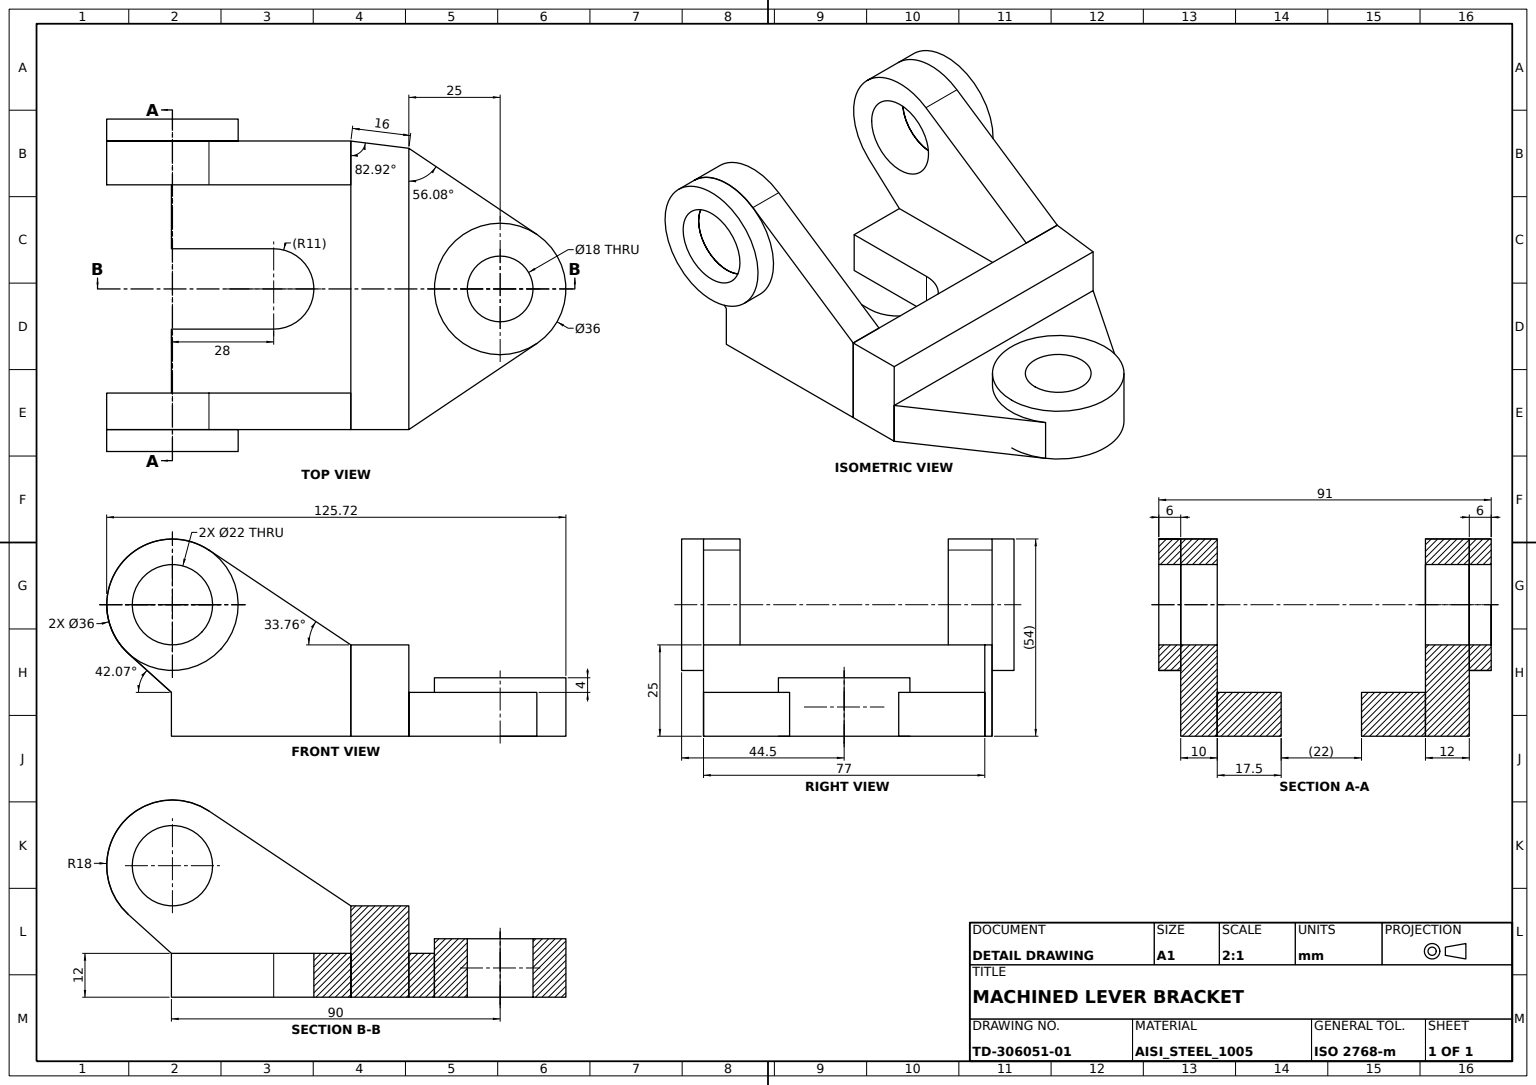
ISO-10303-21;
HEADER;
FILE_DESCRIPTION((''),'2;1');
FILE_NAME('','',(''),(''),'','','');
FILE_SCHEMA(('AUTOMOTIVE_DESIGN'));
ENDSEC;
DATA;
#1=APPLICATION_CONTEXT('');
#2=PRODUCT_CONTEXT('',#1,'mechanical');
#3=PRODUCT('','','',(#2));
#4=PRODUCT_DEFINITION_FORMATION('','',#3);
#5=PRODUCT_DEFINITION_CONTEXT('',#1,'design');
#6=PRODUCT_DEFINITION('','',#4,#5);
#7=PRODUCT_DEFINITION_SHAPE('','',#6);
#8=(LENGTH_UNIT()NAMED_UNIT(*)SI_UNIT(.MILLI.,.METRE.));
#9=(NAMED_UNIT(*)PLANE_ANGLE_UNIT()SI_UNIT($,.RADIAN.));
#10=(NAMED_UNIT(*)SI_UNIT($,.STERADIAN.)SOLID_ANGLE_UNIT());
#11=UNCERTAINTY_MEASURE_WITH_UNIT(LENGTH_MEASURE(0.005),#8,'distance_accuracy_value','');
#12=(GEOMETRIC_REPRESENTATION_CONTEXT(3)GLOBAL_UNCERTAINTY_ASSIGNED_CONTEXT((#11))GLOBAL_UNIT_ASSIGNED_CONTEXT((#8,#9,#10))REPRESENTATION_CONTEXT('',''));
#13=CARTESIAN_POINT('',(-28.5,-40.877865,-8.));
#14=VERTEX_POINT('',#13);
#15=CARTESIAN_POINT('',(-28.5,-90.,-8.));
#16=VERTEX_POINT('',#15);
#17=DIRECTION('',(0.,-1.,0.));
#18=VECTOR('',#17,1000.);
#19=LINE('',#13,#18);
#20=EDGE_CURVE('',#14,#16,#19,.T.);
#21=ORIENTED_EDGE('',*,*,#20,.T.);
#22=CARTESIAN_POINT('',(-40.5,-90.,-8.));
#23=VERTEX_POINT('',#22);
#24=DIRECTION('',(1.,0.,0.));
#25=VECTOR('',#24,1000.);
#26=LINE('',#22,#25);
#27=EDGE_CURVE('',#23,#16,#26,.T.);
#28=ORIENTED_EDGE('',*,*,#27,.F.);
#29=CARTESIAN_POINT('',(-40.5,-40.877865,-8.));
#30=VERTEX_POINT('',#29);
#31=LINE('',#29,#18);
#32=EDGE_CURVE('',#30,#23,#31,.T.);
#33=ORIENTED_EDGE('',*,*,#32,.F.);
#34=LINE('',#29,#25);
#35=EDGE_CURVE('',#30,#14,#34,.T.);
#36=ORIENTED_EDGE('',*,*,#35,.T.);
#37=EDGE_LOOP('',(#21,#28,#33,#36));
#38=FACE_BOUND('',#37,.T.);
#39=DIRECTION('',(0.,0.,1.));
#40=AXIS2_PLACEMENT_3D('',#29,#39,#17);
#41=PLANE('',#40);
#42=ADVANCED_FACE('',(#38),#41,.F.);
#43=CARTESIAN_POINT('',(-40.5,-90.,4.));
#44=VERTEX_POINT('',#43);
#45=VECTOR('',#39,1000.);
#46=LINE('',#22,#45);
#47=EDGE_CURVE('',#23,#44,#46,.T.);
#48=ORIENTED_EDGE('',*,*,#47,.F.);
#49=ORIENTED_EDGE('',*,*,#27,.T.);
#50=CARTESIAN_POINT('',(-28.5,-90.,4.));
#51=VERTEX_POINT('',#50);
#52=LINE('',#15,#45);
#53=EDGE_CURVE('',#16,#51,#52,.T.);
#54=ORIENTED_EDGE('',*,*,#53,.T.);
#55=LINE('',#43,#25);
#56=EDGE_CURVE('',#44,#51,#55,.T.);
#57=ORIENTED_EDGE('',*,*,#56,.F.);
#58=EDGE_LOOP('',(#48,#49,#54,#57));
#59=FACE_BOUND('',#58,.T.);
#60=DIRECTION('',(0.,1.,0.));
#61=AXIS2_PLACEMENT_3D('',#22,#60,#39);
#62=PLANE('',#61);
#63=ADVANCED_FACE('',(#59),#62,.F.);
#64=ORIENTED_EDGE('',*,*,#53,.F.);
#65=ORIENTED_EDGE('',*,*,#20,.F.);
#66=CARTESIAN_POINT('',(-28.5,-40.877865,17.));
#67=VERTEX_POINT('',#66);
#68=DIRECTION('',(0.,0.,-1.));
#69=VECTOR('',#68,1000.);
#70=LINE('',#66,#69);
#71=EDGE_CURVE('',#67,#14,#70,.T.);
#72=ORIENTED_EDGE('',*,*,#71,.F.);
#73=CARTESIAN_POINT('',(-28.5,-79.720085,42.964502));
#74=VERTEX_POINT('',#73);
#75=DIRECTION('',(0.,0.831361229,-0.555732406));
#76=VECTOR('',#75,1000.);
#77=LINE('',#73,#76);
#78=EDGE_CURVE('',#74,#67,#77,.T.);
#79=ORIENTED_EDGE('',*,*,#78,.F.);
#80=CARTESIAN_POINT('',(-28.5,-101.785016,14.639078));
#81=VERTEX_POINT('',#80);
#82=CARTESIAN_POINT('',(-28.5,-89.723268,28.));
#83=DIRECTION('',(-1.,0.,0.));
#84=AXIS2_PLACEMENT_3D('',#82,#83,#17);
#85=CIRCLE('',#84,18.);
#86=EDGE_CURVE('',#81,#74,#85,.T.);
#87=ORIENTED_EDGE('',*,*,#86,.F.);
#88=DIRECTION('',(0.,-0.742273459,0.670097092));
#89=VECTOR('',#88,1000.);
#90=LINE('',#50,#89);
#91=EDGE_CURVE('',#51,#81,#90,.T.);
#92=ORIENTED_EDGE('',*,*,#91,.F.);
#93=EDGE_LOOP('',(#64,#65,#72,#79,#87,#92));
#94=FACE_BOUND('',#93,.T.);
#95=CARTESIAN_POINT('',(-28.5,-100.723268,28.));
#96=VERTEX_POINT('',#95);
#97=AXIS2_PLACEMENT_3D('',#82,#24,#17);
#98=CIRCLE('',#97,11.);
#99=EDGE_CURVE('',#96,#96,#98,.T.);
#100=ORIENTED_EDGE('',*,*,#99,.F.);
#101=EDGE_LOOP('',(#100));
#102=FACE_BOUND('',#101,.T.);
#103=AXIS2_PLACEMENT_3D('',#82,#83,#39);
#104=PLANE('',#103);
#105=ADVANCED_FACE('',(#94,#102),#104,.F.);
#106=ORIENTED_EDGE('',*,*,#99,.T.);
#107=EDGE_LOOP('',(#106));
#108=FACE_BOUND('',#107,.T.);
#109=CARTESIAN_POINT('',(-40.5,-100.723268,28.));
#110=VERTEX_POINT('',#109);
#111=CARTESIAN_POINT('',(-40.5,-89.723268,28.));
#112=AXIS2_PLACEMENT_3D('',#111,#24,#17);
#113=CIRCLE('',#112,11.);
#114=EDGE_CURVE('',#110,#110,#113,.T.);
#115=ORIENTED_EDGE('',*,*,#114,.F.);
#116=EDGE_LOOP('',(#115));
#117=FACE_BOUND('',#116,.T.);
#118=AXIS2_PLACEMENT_3D('',#111,#24,#68);
#119=CYLINDRICAL_SURFACE('',#118,11.);
#120=ADVANCED_FACE('',(#108,#117),#119,.F.);
#121=ORIENTED_EDGE('',*,*,#114,.T.);
#122=EDGE_LOOP('',(#121));
#123=FACE_BOUND('',#122,.T.);
#124=CARTESIAN_POINT('',(-40.5,-101.785016,14.639078));
#125=VERTEX_POINT('',#124);
#126=CARTESIAN_POINT('',(-40.5,-79.720085,42.964502));
#127=VERTEX_POINT('',#126);
#128=AXIS2_PLACEMENT_3D('',#111,#83,#17);
#129=CIRCLE('',#128,18.);
#130=EDGE_CURVE('',#125,#127,#129,.T.);
#131=ORIENTED_EDGE('',*,*,#130,.T.);
#132=CARTESIAN_POINT('',(-40.5,-40.877865,17.));
#133=VERTEX_POINT('',#132);
#134=LINE('',#126,#76);
#135=EDGE_CURVE('',#127,#133,#134,.T.);
#136=ORIENTED_EDGE('',*,*,#135,.T.);
#137=LINE('',#132,#69);
#138=EDGE_CURVE('',#133,#30,#137,.T.);
#139=ORIENTED_EDGE('',*,*,#138,.T.);
#140=ORIENTED_EDGE('',*,*,#32,.T.);
#141=ORIENTED_EDGE('',*,*,#47,.T.);
#142=LINE('',#43,#89);
#143=EDGE_CURVE('',#44,#125,#142,.T.);
#144=ORIENTED_EDGE('',*,*,#143,.T.);
#145=EDGE_LOOP('',(#131,#136,#139,#140,#141,#144));
#146=FACE_BOUND('',#145,.T.);
#147=AXIS2_PLACEMENT_3D('',#111,#83,#39);
#148=PLANE('',#147);
#149=ADVANCED_FACE('',(#123,#146),#148,.T.);
#150=ORIENTED_EDGE('',*,*,#71,.T.);
#151=ORIENTED_EDGE('',*,*,#35,.F.);
#152=ORIENTED_EDGE('',*,*,#138,.F.);
#153=LINE('',#132,#25);
#154=EDGE_CURVE('',#133,#67,#153,.T.);
#155=ORIENTED_EDGE('',*,*,#154,.T.);
#156=EDGE_LOOP('',(#150,#151,#152,#155));
#157=FACE_BOUND('',#156,.T.);
#158=AXIS2_PLACEMENT_3D('',#132,#17,#68);
#159=PLANE('',#158);
#160=ADVANCED_FACE('',(#157),#159,.F.);
#161=LINE('',#124,#25);
#162=EDGE_CURVE('',#125,#81,#161,.T.);
#163=ORIENTED_EDGE('',*,*,#162,.T.);
#164=ORIENTED_EDGE('',*,*,#86,.T.);
#165=LINE('',#126,#25);
#166=EDGE_CURVE('',#127,#74,#165,.T.);
#167=ORIENTED_EDGE('',*,*,#166,.F.);
#168=ORIENTED_EDGE('',*,*,#130,.F.);
#169=EDGE_LOOP('',(#163,#164,#167,#168));
#170=FACE_BOUND('',#169,.T.);
#171=CYLINDRICAL_SURFACE('',#118,18.);
#172=ADVANCED_FACE('',(#170),#171,.T.);
#173=ORIENTED_EDGE('',*,*,#143,.F.);
#174=ORIENTED_EDGE('',*,*,#56,.T.);
#175=ORIENTED_EDGE('',*,*,#91,.T.);
#176=ORIENTED_EDGE('',*,*,#162,.F.);
#177=EDGE_LOOP('',(#173,#174,#175,#176));
#178=FACE_BOUND('',#177,.T.);
#179=DIRECTION('',(0.,0.670097092,0.742273459));
#180=AXIS2_PLACEMENT_3D('',#43,#179,#88);
#181=PLANE('',#180);
#182=ADVANCED_FACE('',(#178),#181,.F.);
#183=ORIENTED_EDGE('',*,*,#135,.F.);
#184=ORIENTED_EDGE('',*,*,#166,.T.);
#185=ORIENTED_EDGE('',*,*,#78,.T.);
#186=ORIENTED_EDGE('',*,*,#154,.F.);
#187=EDGE_LOOP('',(#183,#184,#185,#186));
#188=FACE_BOUND('',#187,.T.);
#189=DIRECTION('',(0.,-0.555732406,-0.831361229));
#190=AXIS2_PLACEMENT_3D('',#126,#189,#75);
#191=PLANE('',#190);
#192=ADVANCED_FACE('',(#188),#191,.F.);
#193=CLOSED_SHELL('',(#42,#63,#105,#120,#149,#160,#172,#182,#192));
#194=MANIFOLD_SOLID_BREP('',#193);
#195=CARTESIAN_POINT('',(38.5,-78.723268,28.));
#196=VERTEX_POINT('',#195);
#197=CARTESIAN_POINT('',(38.5,-89.723268,28.));
#198=AXIS2_PLACEMENT_3D('',#197,#83,#60);
#199=CIRCLE('',#198,11.);
#200=EDGE_CURVE('',#196,#196,#199,.T.);
#201=ORIENTED_EDGE('',*,*,#200,.F.);
#202=EDGE_LOOP('',(#201));
#203=FACE_BOUND('',#202,.T.);
#204=CARTESIAN_POINT('',(28.5,-78.723268,28.));
#205=VERTEX_POINT('',#204);
#206=CARTESIAN_POINT('',(28.5,-89.723268,28.));
#207=AXIS2_PLACEMENT_3D('',#206,#83,#60);
#208=CIRCLE('',#207,11.);
#209=EDGE_CURVE('',#205,#205,#208,.T.);
#210=ORIENTED_EDGE('',*,*,#209,.T.);
#211=EDGE_LOOP('',(#210));
#212=FACE_BOUND('',#211,.T.);
#213=AXIS2_PLACEMENT_3D('',#197,#83,#39);
#214=CYLINDRICAL_SURFACE('',#213,11.);
#215=ADVANCED_FACE('',(#203,#212),#214,.F.);
#216=CARTESIAN_POINT('',(28.5,-90.,-8.));
#217=VERTEX_POINT('',#216);
#218=CARTESIAN_POINT('',(28.5,-40.877865,-8.));
#219=VERTEX_POINT('',#218);
#220=VECTOR('',#60,1000.);
#221=LINE('',#216,#220);
#222=EDGE_CURVE('',#217,#219,#221,.T.);
#223=ORIENTED_EDGE('',*,*,#222,.T.);
#224=CARTESIAN_POINT('',(38.5,-40.877865,-8.));
#225=VERTEX_POINT('',#224);
#226=VECTOR('',#83,1000.);
#227=LINE('',#224,#226);
#228=EDGE_CURVE('',#225,#219,#227,.T.);
#229=ORIENTED_EDGE('',*,*,#228,.F.);
#230=CARTESIAN_POINT('',(38.5,-90.,-8.));
#231=VERTEX_POINT('',#230);
#232=LINE('',#230,#220);
#233=EDGE_CURVE('',#231,#225,#232,.T.);
#234=ORIENTED_EDGE('',*,*,#233,.F.);
#235=LINE('',#230,#226);
#236=EDGE_CURVE('',#231,#217,#235,.T.);
#237=ORIENTED_EDGE('',*,*,#236,.T.);
#238=EDGE_LOOP('',(#223,#229,#234,#237));
#239=FACE_BOUND('',#238,.T.);
#240=AXIS2_PLACEMENT_3D('',#230,#39,#24);
#241=PLANE('',#240);
#242=ADVANCED_FACE('',(#239),#241,.F.);
#243=CARTESIAN_POINT('',(28.5,-40.877865,17.));
#244=VERTEX_POINT('',#243);
#245=CARTESIAN_POINT('',(28.5,-79.720085,42.964502));
#246=VERTEX_POINT('',#245);
#247=DIRECTION('',(0.,-0.831361229,0.555732406));
#248=VECTOR('',#247,1000.);
#249=LINE('',#243,#248);
#250=EDGE_CURVE('',#244,#246,#249,.T.);
#251=ORIENTED_EDGE('',*,*,#250,.T.);
#252=CARTESIAN_POINT('',(38.5,-79.720085,42.964502));
#253=VERTEX_POINT('',#252);
#254=LINE('',#252,#226);
#255=EDGE_CURVE('',#253,#246,#254,.T.);
#256=ORIENTED_EDGE('',*,*,#255,.F.);
#257=CARTESIAN_POINT('',(38.5,-40.877865,17.));
#258=VERTEX_POINT('',#257);
#259=LINE('',#257,#248);
#260=EDGE_CURVE('',#258,#253,#259,.T.);
#261=ORIENTED_EDGE('',*,*,#260,.F.);
#262=LINE('',#257,#226);
#263=EDGE_CURVE('',#258,#244,#262,.T.);
#264=ORIENTED_EDGE('',*,*,#263,.T.);
#265=EDGE_LOOP('',(#251,#256,#261,#264));
#266=FACE_BOUND('',#265,.T.);
#267=AXIS2_PLACEMENT_3D('',#257,#189,#75);
#268=PLANE('',#267);
#269=ADVANCED_FACE('',(#266),#268,.F.);
#270=LINE('',#224,#45);
#271=EDGE_CURVE('',#225,#258,#270,.T.);
#272=ORIENTED_EDGE('',*,*,#271,.F.);
#273=ORIENTED_EDGE('',*,*,#228,.T.);
#274=CARTESIAN_POINT('',(28.5,-40.877865,4.));
#275=LINE('',#274,#45);
#276=EDGE_CURVE('',#219,#244,#275,.T.);
#277=ORIENTED_EDGE('',*,*,#276,.T.);
#278=ORIENTED_EDGE('',*,*,#263,.F.);
#279=EDGE_LOOP('',(#272,#273,#277,#278));
#280=FACE_BOUND('',#279,.T.);
#281=CARTESIAN_POINT('',(38.5,-40.877865,4.));
#282=AXIS2_PLACEMENT_3D('',#281,#17,#68);
#283=PLANE('',#282);
#284=ADVANCED_FACE('',(#280),#283,.F.);
#285=CARTESIAN_POINT('',(28.5,-101.785016,14.639078));
#286=VERTEX_POINT('',#285);
#287=AXIS2_PLACEMENT_3D('',#206,#24,#60);
#288=CIRCLE('',#287,18.);
#289=EDGE_CURVE('',#246,#286,#288,.T.);
#290=ORIENTED_EDGE('',*,*,#289,.T.);
#291=CARTESIAN_POINT('',(38.5,-101.785016,14.639078));
#292=VERTEX_POINT('',#291);
#293=LINE('',#291,#226);
#294=EDGE_CURVE('',#292,#286,#293,.T.);
#295=ORIENTED_EDGE('',*,*,#294,.F.);
#296=AXIS2_PLACEMENT_3D('',#197,#24,#60);
#297=CIRCLE('',#296,18.);
#298=EDGE_CURVE('',#253,#292,#297,.T.);
#299=ORIENTED_EDGE('',*,*,#298,.F.);
#300=ORIENTED_EDGE('',*,*,#255,.T.);
#301=EDGE_LOOP('',(#290,#295,#299,#300));
#302=FACE_BOUND('',#301,.T.);
#303=CYLINDRICAL_SURFACE('',#213,18.);
#304=ADVANCED_FACE('',(#302),#303,.T.);
#305=ORIENTED_EDGE('',*,*,#236,.F.);
#306=CARTESIAN_POINT('',(38.5,-90.,4.));
#307=VERTEX_POINT('',#306);
#308=LINE('',#306,#69);
#309=EDGE_CURVE('',#307,#231,#308,.T.);
#310=ORIENTED_EDGE('',*,*,#309,.F.);
#311=CARTESIAN_POINT('',(28.5,-90.,4.));
#312=VERTEX_POINT('',#311);
#313=LINE('',#306,#226);
#314=EDGE_CURVE('',#307,#312,#313,.T.);
#315=ORIENTED_EDGE('',*,*,#314,.T.);
#316=LINE('',#311,#69);
#317=EDGE_CURVE('',#312,#217,#316,.T.);
#318=ORIENTED_EDGE('',*,*,#317,.T.);
#319=EDGE_LOOP('',(#305,#310,#315,#318));
#320=FACE_BOUND('',#319,.T.);
#321=AXIS2_PLACEMENT_3D('',#306,#60,#39);
#322=PLANE('',#321);
#323=ADVANCED_FACE('',(#320),#322,.F.);
#324=ORIENTED_EDGE('',*,*,#200,.T.);
#325=EDGE_LOOP('',(#324));
#326=FACE_BOUND('',#325,.T.);
#327=ORIENTED_EDGE('',*,*,#271,.T.);
#328=ORIENTED_EDGE('',*,*,#260,.T.);
#329=ORIENTED_EDGE('',*,*,#298,.T.);
#330=DIRECTION('',(0.,0.742273459,-0.670097092));
#331=VECTOR('',#330,1000.);
#332=LINE('',#291,#331);
#333=EDGE_CURVE('',#292,#307,#332,.T.);
#334=ORIENTED_EDGE('',*,*,#333,.T.);
#335=ORIENTED_EDGE('',*,*,#309,.T.);
#336=ORIENTED_EDGE('',*,*,#233,.T.);
#337=EDGE_LOOP('',(#327,#328,#329,#334,#335,#336));
#338=FACE_BOUND('',#337,.T.);
#339=AXIS2_PLACEMENT_3D('',#197,#24,#68);
#340=PLANE('',#339);
#341=ADVANCED_FACE('',(#326,#338),#340,.T.);
#342=ORIENTED_EDGE('',*,*,#209,.F.);
#343=EDGE_LOOP('',(#342));
#344=FACE_BOUND('',#343,.T.);
#345=ORIENTED_EDGE('',*,*,#250,.F.);
#346=ORIENTED_EDGE('',*,*,#276,.F.);
#347=ORIENTED_EDGE('',*,*,#222,.F.);
#348=ORIENTED_EDGE('',*,*,#317,.F.);
#349=LINE('',#285,#331);
#350=EDGE_CURVE('',#286,#312,#349,.T.);
#351=ORIENTED_EDGE('',*,*,#350,.F.);
#352=ORIENTED_EDGE('',*,*,#289,.F.);
#353=EDGE_LOOP('',(#345,#346,#347,#348,#351,#352));
#354=FACE_BOUND('',#353,.T.);
#355=AXIS2_PLACEMENT_3D('',#206,#24,#68);
#356=PLANE('',#355);
#357=ADVANCED_FACE('',(#344,#354),#356,.F.);
#358=ORIENTED_EDGE('',*,*,#350,.T.);
#359=ORIENTED_EDGE('',*,*,#314,.F.);
#360=ORIENTED_EDGE('',*,*,#333,.F.);
#361=ORIENTED_EDGE('',*,*,#294,.T.);
#362=EDGE_LOOP('',(#358,#359,#360,#361));
#363=FACE_BOUND('',#362,.T.);
#364=AXIS2_PLACEMENT_3D('',#291,#179,#88);
#365=PLANE('',#364);
#366=ADVANCED_FACE('',(#363),#365,.F.);
#367=CLOSED_SHELL('',(#215,#242,#269,#284,#304,#323,#341,#357,#366));
#368=MANIFOLD_SOLID_BREP('',#367);
#369=CARTESIAN_POINT('',(38.5,-25.,17.));
#370=VERTEX_POINT('',#369);
#371=VERTEX_POINT('',#257);
#372=LINE('',#369,#18);
#373=EDGE_CURVE('',#370,#371,#372,.T.);
#374=ORIENTED_EDGE('',*,*,#373,.T.);
#375=VERTEX_POINT('',#224);
#376=LINE('',#257,#69);
#377=EDGE_CURVE('',#371,#375,#376,.T.);
#378=ORIENTED_EDGE('',*,*,#377,.T.);
#379=CARTESIAN_POINT('',(38.5,-25.,-8.));
#380=VERTEX_POINT('',#379);
#381=LINE('',#379,#18);
#382=EDGE_CURVE('',#380,#375,#381,.T.);
#383=ORIENTED_EDGE('',*,*,#382,.F.);
#384=LINE('',#369,#69);
#385=EDGE_CURVE('',#370,#380,#384,.T.);
#386=ORIENTED_EDGE('',*,*,#385,.F.);
#387=EDGE_LOOP('',(#374,#378,#383,#386));
#388=FACE_BOUND('',#387,.T.);
#389=AXIS2_PLACEMENT_3D('',#369,#24,#60);
#390=PLANE('',#389);
#391=ADVANCED_FACE('',(#388),#390,.T.);
#392=CARTESIAN_POINT('',(-40.47317,-40.877865,-8.));
#393=VERTEX_POINT('',#392);
#394=EDGE_CURVE('',#375,#393,#227,.T.);
#395=ORIENTED_EDGE('',*,*,#394,.F.);
#396=ORIENTED_EDGE('',*,*,#377,.F.);
#397=CARTESIAN_POINT('',(-40.47317,-40.877865,17.));
#398=VERTEX_POINT('',#397);
#399=EDGE_CURVE('',#371,#398,#262,.T.);
#400=ORIENTED_EDGE('',*,*,#399,.T.);
#401=LINE('',#397,#69);
#402=EDGE_CURVE('',#398,#393,#401,.T.);
#403=ORIENTED_EDGE('',*,*,#402,.T.);
#404=EDGE_LOOP('',(#395,#396,#400,#403));
#405=FACE_BOUND('',#404,.T.);
#406=AXIS2_PLACEMENT_3D('',#257,#17,#24);
#407=PLANE('',#406);
#408=ADVANCED_FACE('',(#405),#407,.T.);
#409=ORIENTED_EDGE('',*,*,#382,.T.);
#410=ORIENTED_EDGE('',*,*,#394,.T.);
#411=CARTESIAN_POINT('',(-38.5,-25.,-8.));
#412=VERTEX_POINT('',#411);
#413=DIRECTION('',(0.123323103,0.992366572,0.));
#414=VECTOR('',#413,1000.);
#415=LINE('',#392,#414);
#416=EDGE_CURVE('',#393,#412,#415,.T.);
#417=ORIENTED_EDGE('',*,*,#416,.T.);
#418=LINE('',#411,#25);
#419=EDGE_CURVE('',#412,#380,#418,.T.);
#420=ORIENTED_EDGE('',*,*,#419,.T.);
#421=EDGE_LOOP('',(#409,#410,#417,#420));
#422=FACE_BOUND('',#421,.T.);
#423=CARTESIAN_POINT('',(0.,0.,-8.));
#424=AXIS2_PLACEMENT_3D('',#423,#39,#24);
#425=PLANE('',#424);
#426=ADVANCED_FACE('',(#422),#425,.F.);
#427=CARTESIAN_POINT('',(-38.5,-25.,17.));
#428=VERTEX_POINT('',#427);
#429=LINE('',#427,#69);
#430=EDGE_CURVE('',#428,#412,#429,.T.);
#431=ORIENTED_EDGE('',*,*,#430,.F.);
#432=LINE('',#427,#25);
#433=EDGE_CURVE('',#428,#370,#432,.T.);
#434=ORIENTED_EDGE('',*,*,#433,.T.);
#435=ORIENTED_EDGE('',*,*,#385,.T.);
#436=ORIENTED_EDGE('',*,*,#419,.F.);
#437=EDGE_LOOP('',(#431,#434,#435,#436));
#438=FACE_BOUND('',#437,.T.);
#439=AXIS2_PLACEMENT_3D('',#427,#60,#83);
#440=PLANE('',#439);
#441=ADVANCED_FACE('',(#438),#440,.T.);
#442=ORIENTED_EDGE('',*,*,#416,.F.);
#443=ORIENTED_EDGE('',*,*,#402,.F.);
#444=LINE('',#397,#414);
#445=EDGE_CURVE('',#398,#428,#444,.T.);
#446=ORIENTED_EDGE('',*,*,#445,.T.);
#447=ORIENTED_EDGE('',*,*,#430,.T.);
#448=EDGE_LOOP('',(#442,#443,#446,#447));
#449=FACE_BOUND('',#448,.T.);
#450=DIRECTION('',(-0.992366572,0.123323103,0.));
#451=DIRECTION('',(-0.123323103,-0.992366572,0.));
#452=AXIS2_PLACEMENT_3D('',#397,#450,#451);
#453=PLANE('',#452);
#454=ADVANCED_FACE('',(#449),#453,.T.);
#455=ORIENTED_EDGE('',*,*,#445,.F.);
#456=ORIENTED_EDGE('',*,*,#399,.F.);
#457=ORIENTED_EDGE('',*,*,#373,.F.);
#458=ORIENTED_EDGE('',*,*,#433,.F.);
#459=EDGE_LOOP('',(#455,#456,#457,#458));
#460=FACE_BOUND('',#459,.T.);
#461=CARTESIAN_POINT('',(0.,0.,17.));
#462=AXIS2_PLACEMENT_3D('',#461,#39,#24);
#463=PLANE('',#462);
#464=ADVANCED_FACE('',(#460),#463,.T.);
#465=CLOSED_SHELL('',(#391,#408,#426,#441,#454,#464));
#466=MANIFOLD_SOLID_BREP('',#465);
#467=CARTESIAN_POINT('',(38.5,-25.,4.));
#468=VERTEX_POINT('',#467);
#469=CARTESIAN_POINT('',(-38.5,-25.,4.));
#470=VERTEX_POINT('',#469);
#471=LINE('',#469,#25);
#472=EDGE_CURVE('',#468,#470,#471,.F.);
#473=ORIENTED_EDGE('',*,*,#472,.T.);
#474=VERTEX_POINT('',#411);
#475=LINE('',#469,#69);
#476=EDGE_CURVE('',#474,#470,#475,.F.);
#477=ORIENTED_EDGE('',*,*,#476,.F.);
#478=VERTEX_POINT('',#379);
#479=EDGE_CURVE('',#478,#474,#418,.F.);
#480=ORIENTED_EDGE('',*,*,#479,.F.);
#481=LINE('',#467,#69);
#482=EDGE_CURVE('',#478,#468,#481,.F.);
#483=ORIENTED_EDGE('',*,*,#482,.T.);
#484=EDGE_LOOP('',(#473,#477,#480,#483));
#485=FACE_BOUND('',#484,.T.);
#486=AXIS2_PLACEMENT_3D('',#469,#60,#39);
#487=PLANE('',#486);
#488=ADVANCED_FACE('',(#485),#487,.F.);
#489=CARTESIAN_POINT('',(-14.937404,10.043603,-8.));
#490=VERTEX_POINT('',#489);
#491=DIRECTION('',(-0.557977922,-0.829855794,0.));
#492=VECTOR('',#491,1000.);
#493=LINE('',#489,#492);
#494=EDGE_CURVE('',#474,#490,#493,.F.);
#495=ORIENTED_EDGE('',*,*,#494,.F.);
#496=ORIENTED_EDGE('',*,*,#476,.T.);
#497=CARTESIAN_POINT('',(-14.937404,10.043603,4.));
#498=VERTEX_POINT('',#497);
#499=LINE('',#497,#492);
#500=EDGE_CURVE('',#470,#498,#499,.F.);
#501=ORIENTED_EDGE('',*,*,#500,.T.);
#502=LINE('',#497,#69);
#503=EDGE_CURVE('',#490,#498,#502,.F.);
#504=ORIENTED_EDGE('',*,*,#503,.F.);
#505=EDGE_LOOP('',(#495,#496,#501,#504));
#506=FACE_BOUND('',#505,.T.);
#507=DIRECTION('',(0.829855794,-0.557977922,0.));
#508=DIRECTION('',(0.557977922,0.829855794,0.));
#509=AXIS2_PLACEMENT_3D('',#497,#507,#508);
#510=PLANE('',#509);
#511=ADVANCED_FACE('',(#506),#510,.F.);
#512=ORIENTED_EDGE('',*,*,#482,.F.);
#513=CARTESIAN_POINT('',(14.937404,10.043603,-8.));
#514=VERTEX_POINT('',#513);
#515=DIRECTION('',(-0.557977922,0.829855794,0.));
#516=VECTOR('',#515,1000.);
#517=LINE('',#379,#516);
#518=EDGE_CURVE('',#514,#478,#517,.F.);
#519=ORIENTED_EDGE('',*,*,#518,.F.);
#520=CARTESIAN_POINT('',(14.937404,10.043603,4.));
#521=VERTEX_POINT('',#520);
#522=LINE('',#520,#69);
#523=EDGE_CURVE('',#514,#521,#522,.F.);
#524=ORIENTED_EDGE('',*,*,#523,.T.);
#525=LINE('',#467,#516);
#526=EDGE_CURVE('',#521,#468,#525,.F.);
#527=ORIENTED_EDGE('',*,*,#526,.T.);
#528=EDGE_LOOP('',(#512,#519,#524,#527));
#529=FACE_BOUND('',#528,.T.);
#530=DIRECTION('',(-0.829855794,-0.557977922,0.));
#531=DIRECTION('',(0.557977922,-0.829855794,0.));
#532=AXIS2_PLACEMENT_3D('',#467,#530,#531);
#533=PLANE('',#532);
#534=ADVANCED_FACE('',(#529),#533,.F.);
#535=ORIENTED_EDGE('',*,*,#500,.F.);
#536=ORIENTED_EDGE('',*,*,#472,.F.);
#537=ORIENTED_EDGE('',*,*,#526,.F.);
#538=CARTESIAN_POINT('',(0.,0.,4.));
#539=AXIS2_PLACEMENT_3D('',#538,#68,#24);
#540=CIRCLE('',#539,18.);
#541=EDGE_CURVE('',#498,#521,#540,.F.);
#542=ORIENTED_EDGE('',*,*,#541,.F.);
#543=EDGE_LOOP('',(#535,#536,#537,#542));
#544=FACE_BOUND('',#543,.T.);
#545=AXIS2_PLACEMENT_3D('',#538,#68,#83);
#546=PLANE('',#545);
#547=ADVANCED_FACE('',(#544),#546,.F.);
#548=ORIENTED_EDGE('',*,*,#541,.T.);
#549=ORIENTED_EDGE('',*,*,#523,.F.);
#550=AXIS2_PLACEMENT_3D('',#423,#68,#24);
#551=CIRCLE('',#550,18.);
#552=EDGE_CURVE('',#490,#514,#551,.F.);
#553=ORIENTED_EDGE('',*,*,#552,.F.);
#554=ORIENTED_EDGE('',*,*,#503,.T.);
#555=EDGE_LOOP('',(#548,#549,#553,#554));
#556=FACE_BOUND('',#555,.T.);
#557=CYLINDRICAL_SURFACE('',#545,18.);
#558=ADVANCED_FACE('',(#556),#557,.F.);
#559=ORIENTED_EDGE('',*,*,#552,.T.);
#560=ORIENTED_EDGE('',*,*,#518,.T.);
#561=ORIENTED_EDGE('',*,*,#479,.T.);
#562=ORIENTED_EDGE('',*,*,#494,.T.);
#563=EDGE_LOOP('',(#559,#560,#561,#562));
#564=FACE_BOUND('',#563,.T.);
#565=AXIS2_PLACEMENT_3D('',#423,#68,#83);
#566=PLANE('',#565);
#567=ADVANCED_FACE('',(#564),#566,.T.);
#568=CLOSED_SHELL('',(#488,#511,#534,#547,#558,#567));
#569=MANIFOLD_SOLID_BREP('',#568);
#570=CARTESIAN_POINT('',(-11.,-62.,4.));
#571=VERTEX_POINT('',#570);
#572=CARTESIAN_POINT('',(-11.,-90.,4.));
#573=VERTEX_POINT('',#572);
#574=LINE('',#570,#18);
#575=EDGE_CURVE('',#571,#573,#574,.T.);
#576=ORIENTED_EDGE('',*,*,#575,.F.);
#577=CARTESIAN_POINT('',(11.,-62.,4.));
#578=VERTEX_POINT('',#577);
#579=CARTESIAN_POINT('',(0.,-62.,4.));
#580=AXIS2_PLACEMENT_3D('',#579,#39,#83);
#581=CIRCLE('',#580,11.);
#582=EDGE_CURVE('',#578,#571,#581,.T.);
#583=ORIENTED_EDGE('',*,*,#582,.F.);
#584=CARTESIAN_POINT('',(11.,-90.,4.));
#585=VERTEX_POINT('',#584);
#586=LINE('',#584,#220);
#587=EDGE_CURVE('',#585,#578,#586,.T.);
#588=ORIENTED_EDGE('',*,*,#587,.F.);
#589=VERTEX_POINT('',#311);
#590=LINE('',#311,#226);
#591=EDGE_CURVE('',#589,#585,#590,.T.);
#592=ORIENTED_EDGE('',*,*,#591,.F.);
#593=VERTEX_POINT('',#274);
#594=LINE('',#274,#18);
#595=EDGE_CURVE('',#593,#589,#594,.T.);
#596=ORIENTED_EDGE('',*,*,#595,.F.);
#597=CARTESIAN_POINT('',(-28.5,-40.877865,4.));
#598=VERTEX_POINT('',#597);
#599=LINE('',#597,#25);
#600=EDGE_CURVE('',#598,#593,#599,.T.);
#601=ORIENTED_EDGE('',*,*,#600,.F.);
#602=VERTEX_POINT('',#50);
#603=LINE('',#50,#220);
#604=EDGE_CURVE('',#602,#598,#603,.T.);
#605=ORIENTED_EDGE('',*,*,#604,.F.);
#606=LINE('',#572,#226);
#607=EDGE_CURVE('',#573,#602,#606,.T.);
#608=ORIENTED_EDGE('',*,*,#607,.F.);
#609=EDGE_LOOP('',(#576,#583,#588,#592,#596,#601,#605,#608));
#610=FACE_BOUND('',#609,.T.);
#611=AXIS2_PLACEMENT_3D('',#579,#39,#24);
#612=PLANE('',#611);
#613=ADVANCED_FACE('',(#610),#612,.T.);
#614=VERTEX_POINT('',#216);
#615=CARTESIAN_POINT('',(11.,-90.,-8.));
#616=VERTEX_POINT('',#615);
#617=LINE('',#216,#226);
#618=EDGE_CURVE('',#614,#616,#617,.T.);
#619=ORIENTED_EDGE('',*,*,#618,.F.);
#620=EDGE_CURVE('',#589,#614,#316,.T.);
#621=ORIENTED_EDGE('',*,*,#620,.F.);
#622=ORIENTED_EDGE('',*,*,#591,.T.);
#623=LINE('',#584,#69);
#624=EDGE_CURVE('',#585,#616,#623,.T.);
#625=ORIENTED_EDGE('',*,*,#624,.T.);
#626=EDGE_LOOP('',(#619,#621,#622,#625));
#627=FACE_BOUND('',#626,.T.);
#628=AXIS2_PLACEMENT_3D('',#311,#17,#68);
#629=PLANE('',#628);
#630=ADVANCED_FACE('',(#627),#629,.T.);
#631=ORIENTED_EDGE('',*,*,#600,.T.);
#632=VERTEX_POINT('',#218);
#633=LINE('',#274,#69);
#634=EDGE_CURVE('',#593,#632,#633,.T.);
#635=ORIENTED_EDGE('',*,*,#634,.T.);
#636=VERTEX_POINT('',#13);
#637=LINE('',#13,#25);
#638=EDGE_CURVE('',#636,#632,#637,.T.);
#639=ORIENTED_EDGE('',*,*,#638,.F.);
#640=LINE('',#597,#69);
#641=EDGE_CURVE('',#598,#636,#640,.T.);
#642=ORIENTED_EDGE('',*,*,#641,.F.);
#643=EDGE_LOOP('',(#631,#635,#639,#642));
#644=FACE_BOUND('',#643,.T.);
#645=AXIS2_PLACEMENT_3D('',#597,#60,#83);
#646=PLANE('',#645);
#647=ADVANCED_FACE('',(#644),#646,.T.);
#648=CARTESIAN_POINT('',(11.,-62.,-8.));
#649=VERTEX_POINT('',#648);
#650=LINE('',#577,#69);
#651=EDGE_CURVE('',#578,#649,#650,.T.);
#652=ORIENTED_EDGE('',*,*,#651,.T.);
#653=LINE('',#615,#220);
#654=EDGE_CURVE('',#616,#649,#653,.T.);
#655=ORIENTED_EDGE('',*,*,#654,.F.);
#656=ORIENTED_EDGE('',*,*,#624,.F.);
#657=ORIENTED_EDGE('',*,*,#587,.T.);
#658=EDGE_LOOP('',(#652,#655,#656,#657));
#659=FACE_BOUND('',#658,.T.);
#660=AXIS2_PLACEMENT_3D('',#584,#83,#17);
#661=PLANE('',#660);
#662=ADVANCED_FACE('',(#659),#661,.T.);
#663=CARTESIAN_POINT('',(-11.,-90.,-8.));
#664=VERTEX_POINT('',#663);
#665=VERTEX_POINT('',#15);
#666=LINE('',#663,#226);
#667=EDGE_CURVE('',#664,#665,#666,.T.);
#668=ORIENTED_EDGE('',*,*,#667,.F.);
#669=LINE('',#572,#69);
#670=EDGE_CURVE('',#573,#664,#669,.T.);
#671=ORIENTED_EDGE('',*,*,#670,.F.);
#672=ORIENTED_EDGE('',*,*,#607,.T.);
#673=LINE('',#50,#69);
#674=EDGE_CURVE('',#602,#665,#673,.T.);
#675=ORIENTED_EDGE('',*,*,#674,.T.);
#676=EDGE_LOOP('',(#668,#671,#672,#675));
#677=FACE_BOUND('',#676,.T.);
#678=AXIS2_PLACEMENT_3D('',#572,#17,#68);
#679=PLANE('',#678);
#680=ADVANCED_FACE('',(#677),#679,.T.);
#681=ORIENTED_EDGE('',*,*,#670,.T.);
#682=CARTESIAN_POINT('',(-11.,-62.,-8.));
#683=VERTEX_POINT('',#682);
#684=LINE('',#682,#18);
#685=EDGE_CURVE('',#683,#664,#684,.T.);
#686=ORIENTED_EDGE('',*,*,#685,.F.);
#687=LINE('',#570,#69);
#688=EDGE_CURVE('',#571,#683,#687,.T.);
#689=ORIENTED_EDGE('',*,*,#688,.F.);
#690=ORIENTED_EDGE('',*,*,#575,.T.);
#691=EDGE_LOOP('',(#681,#686,#689,#690));
#692=FACE_BOUND('',#691,.T.);
#693=AXIS2_PLACEMENT_3D('',#570,#24,#68);
#694=PLANE('',#693);
#695=ADVANCED_FACE('',(#692),#694,.T.);
#696=ORIENTED_EDGE('',*,*,#651,.F.);
#697=ORIENTED_EDGE('',*,*,#582,.T.);
#698=ORIENTED_EDGE('',*,*,#688,.T.);
#699=CARTESIAN_POINT('',(0.,-62.,-8.));
#700=AXIS2_PLACEMENT_3D('',#699,#39,#83);
#701=CIRCLE('',#700,11.);
#702=EDGE_CURVE('',#649,#683,#701,.T.);
#703=ORIENTED_EDGE('',*,*,#702,.F.);
#704=EDGE_LOOP('',(#696,#697,#698,#703));
#705=FACE_BOUND('',#704,.T.);
#706=AXIS2_PLACEMENT_3D('',#579,#68,#83);
#707=CYLINDRICAL_SURFACE('',#706,11.);
#708=ADVANCED_FACE('',(#705),#707,.F.);
#709=ORIENTED_EDGE('',*,*,#667,.T.);
#710=LINE('',#15,#220);
#711=EDGE_CURVE('',#665,#636,#710,.T.);
#712=ORIENTED_EDGE('',*,*,#711,.T.);
#713=ORIENTED_EDGE('',*,*,#638,.T.);
#714=LINE('',#218,#18);
#715=EDGE_CURVE('',#632,#614,#714,.T.);
#716=ORIENTED_EDGE('',*,*,#715,.T.);
#717=ORIENTED_EDGE('',*,*,#618,.T.);
#718=ORIENTED_EDGE('',*,*,#654,.T.);
#719=ORIENTED_EDGE('',*,*,#702,.T.);
#720=ORIENTED_EDGE('',*,*,#685,.T.);
#721=EDGE_LOOP('',(#709,#712,#713,#716,#717,#718,#719,#720));
#722=FACE_BOUND('',#721,.T.);
#723=AXIS2_PLACEMENT_3D('',#699,#39,#24);
#724=PLANE('',#723);
#725=ADVANCED_FACE('',(#722),#724,.F.);
#726=ORIENTED_EDGE('',*,*,#715,.F.);
#727=ORIENTED_EDGE('',*,*,#634,.F.);
#728=ORIENTED_EDGE('',*,*,#595,.T.);
#729=ORIENTED_EDGE('',*,*,#620,.T.);
#730=EDGE_LOOP('',(#726,#727,#728,#729));
#731=FACE_BOUND('',#730,.T.);
#732=AXIS2_PLACEMENT_3D('',#274,#24,#68);
#733=PLANE('',#732);
#734=ADVANCED_FACE('',(#731),#733,.T.);
#735=ORIENTED_EDGE('',*,*,#711,.F.);
#736=ORIENTED_EDGE('',*,*,#674,.F.);
#737=ORIENTED_EDGE('',*,*,#604,.T.);
#738=ORIENTED_EDGE('',*,*,#641,.T.);
#739=EDGE_LOOP('',(#735,#736,#737,#738));
#740=FACE_BOUND('',#739,.T.);
#741=AXIS2_PLACEMENT_3D('',#50,#83,#17);
#742=PLANE('',#741);
#743=ADVANCED_FACE('',(#740),#742,.T.);
#744=CLOSED_SHELL('',(#613,#630,#647,#662,#680,#695,#708,#725,#734,#743));
#745=MANIFOLD_SOLID_BREP('',#744);
#746=CARTESIAN_POINT('',(38.5,-81.55826,20.628932));
#747=VERTEX_POINT('',#746);
#748=AXIS2_PLACEMENT_3D('',#197,#83,#330);
#749=CIRCLE('',#748,11.);
#750=EDGE_CURVE('',#747,#747,#749,.T.);
#751=ORIENTED_EDGE('',*,*,#750,.T.);
#752=EDGE_LOOP('',(#751));
#753=FACE_BOUND('',#752,.T.);
#754=CARTESIAN_POINT('',(44.5,-81.55826,20.628932));
#755=VERTEX_POINT('',#754);
#756=CARTESIAN_POINT('',(44.5,-89.723268,28.));
#757=AXIS2_PLACEMENT_3D('',#756,#83,#330);
#758=CIRCLE('',#757,11.);
#759=EDGE_CURVE('',#755,#755,#758,.T.);
#760=ORIENTED_EDGE('',*,*,#759,.F.);
#761=EDGE_LOOP('',(#760));
#762=FACE_BOUND('',#761,.T.);
#763=AXIS2_PLACEMENT_3D('',#756,#83,#39);
#764=CYLINDRICAL_SURFACE('',#763,11.);
#765=ADVANCED_FACE('',(#753,#762),#764,.F.);
#766=CARTESIAN_POINT('',(38.5,-76.362346,15.938252));
#767=VERTEX_POINT('',#766);
#768=CIRCLE('',#748,18.);
#769=EDGE_CURVE('',#767,#767,#768,.T.);
#770=ORIENTED_EDGE('',*,*,#769,.F.);
#771=EDGE_LOOP('',(#770));
#772=FACE_BOUND('',#771,.T.);
#773=CARTESIAN_POINT('',(44.5,-76.362346,15.938252));
#774=VERTEX_POINT('',#773);
#775=CIRCLE('',#757,18.);
#776=EDGE_CURVE('',#774,#774,#775,.T.);
#777=ORIENTED_EDGE('',*,*,#776,.T.);
#778=EDGE_LOOP('',(#777));
#779=FACE_BOUND('',#778,.T.);
#780=CYLINDRICAL_SURFACE('',#763,18.);
#781=ADVANCED_FACE('',(#772,#779),#780,.T.);
#782=ORIENTED_EDGE('',*,*,#759,.T.);
#783=EDGE_LOOP('',(#782));
#784=FACE_BOUND('',#783,.T.);
#785=ORIENTED_EDGE('',*,*,#776,.F.);
#786=EDGE_LOOP('',(#785));
#787=FACE_BOUND('',#786,.T.);
#788=PLANE('',#763);
#789=ADVANCED_FACE('',(#784,#787),#788,.F.);
#790=ORIENTED_EDGE('',*,*,#769,.T.);
#791=EDGE_LOOP('',(#790));
#792=FACE_BOUND('',#791,.T.);
#793=ORIENTED_EDGE('',*,*,#750,.F.);
#794=EDGE_LOOP('',(#793));
#795=FACE_BOUND('',#794,.T.);
#796=PLANE('',#213);
#797=ADVANCED_FACE('',(#792,#795),#796,.T.);
#798=CLOSED_SHELL('',(#765,#781,#789,#797));
#799=MANIFOLD_SOLID_BREP('',#798);
#800=CARTESIAN_POINT('',(18.,0.,8.));
#801=VERTEX_POINT('',#800);
#802=CARTESIAN_POINT('',(0.,0.,8.));
#803=AXIS2_PLACEMENT_3D('',#802,#68,#24);
#804=CIRCLE('',#803,18.);
#805=EDGE_CURVE('',#801,#801,#804,.T.);
#806=ORIENTED_EDGE('',*,*,#805,.F.);
#807=EDGE_LOOP('',(#806));
#808=FACE_BOUND('',#807,.T.);
#809=CARTESIAN_POINT('',(9.,0.,8.));
#810=VERTEX_POINT('',#809);
#811=CIRCLE('',#803,9.);
#812=EDGE_CURVE('',#810,#810,#811,.T.);
#813=ORIENTED_EDGE('',*,*,#812,.T.);
#814=EDGE_LOOP('',(#813));
#815=FACE_BOUND('',#814,.T.);
#816=AXIS2_PLACEMENT_3D('',#802,#68,#83);
#817=PLANE('',#816);
#818=ADVANCED_FACE('',(#808,#815),#817,.F.);
#819=ORIENTED_EDGE('',*,*,#805,.T.);
#820=EDGE_LOOP('',(#819));
#821=FACE_BOUND('',#820,.T.);
#822=CARTESIAN_POINT('',(18.,0.,-8.));
#823=VERTEX_POINT('',#822);
#824=EDGE_CURVE('',#823,#823,#551,.T.);
#825=ORIENTED_EDGE('',*,*,#824,.F.);
#826=EDGE_LOOP('',(#825));
#827=FACE_BOUND('',#826,.T.);
#828=CYLINDRICAL_SURFACE('',#816,18.);
#829=ADVANCED_FACE('',(#821,#827),#828,.T.);
#830=ORIENTED_EDGE('',*,*,#812,.F.);
#831=EDGE_LOOP('',(#830));
#832=FACE_BOUND('',#831,.T.);
#833=CARTESIAN_POINT('',(9.,0.,-8.));
#834=VERTEX_POINT('',#833);
#835=CIRCLE('',#550,9.);
#836=EDGE_CURVE('',#834,#834,#835,.T.);
#837=ORIENTED_EDGE('',*,*,#836,.T.);
#838=EDGE_LOOP('',(#837));
#839=FACE_BOUND('',#838,.T.);
#840=CYLINDRICAL_SURFACE('',#816,9.);
#841=ADVANCED_FACE('',(#832,#839),#840,.F.);
#842=ORIENTED_EDGE('',*,*,#836,.F.);
#843=EDGE_LOOP('',(#842));
#844=FACE_BOUND('',#843,.T.);
#845=ORIENTED_EDGE('',*,*,#824,.T.);
#846=EDGE_LOOP('',(#845));
#847=FACE_BOUND('',#846,.T.);
#848=ADVANCED_FACE('',(#844,#847),#566,.T.);
#849=CLOSED_SHELL('',(#818,#829,#841,#848));
#850=MANIFOLD_SOLID_BREP('',#849);
#851=CARTESIAN_POINT('',(-40.5,-107.723268,28.));
#852=VERTEX_POINT('',#851);
#853=CIRCLE('',#112,18.);
#854=EDGE_CURVE('',#852,#852,#853,.T.);
#855=ORIENTED_EDGE('',*,*,#854,.T.);
#856=EDGE_LOOP('',(#855));
#857=FACE_BOUND('',#856,.T.);
#858=VERTEX_POINT('',#109);
#859=EDGE_CURVE('',#858,#858,#113,.T.);
#860=ORIENTED_EDGE('',*,*,#859,.F.);
#861=EDGE_LOOP('',(#860));
#862=FACE_BOUND('',#861,.T.);
#863=PLANE('',#118);
#864=ADVANCED_FACE('',(#857,#862),#863,.T.);
#865=CARTESIAN_POINT('',(-46.5,-100.723268,28.));
#866=VERTEX_POINT('',#865);
#867=CARTESIAN_POINT('',(-46.5,-89.723268,28.));
#868=AXIS2_PLACEMENT_3D('',#867,#24,#17);
#869=CIRCLE('',#868,11.);
#870=EDGE_CURVE('',#866,#866,#869,.T.);
#871=ORIENTED_EDGE('',*,*,#870,.T.);
#872=EDGE_LOOP('',(#871));
#873=FACE_BOUND('',#872,.T.);
#874=CARTESIAN_POINT('',(-46.5,-107.723268,28.));
#875=VERTEX_POINT('',#874);
#876=CIRCLE('',#868,18.);
#877=EDGE_CURVE('',#875,#875,#876,.T.);
#878=ORIENTED_EDGE('',*,*,#877,.F.);
#879=EDGE_LOOP('',(#878));
#880=FACE_BOUND('',#879,.T.);
#881=AXIS2_PLACEMENT_3D('',#867,#24,#68);
#882=PLANE('',#881);
#883=ADVANCED_FACE('',(#873,#880),#882,.F.);
#884=ORIENTED_EDGE('',*,*,#870,.F.);
#885=EDGE_LOOP('',(#884));
#886=FACE_BOUND('',#885,.T.);
#887=ORIENTED_EDGE('',*,*,#859,.T.);
#888=EDGE_LOOP('',(#887));
#889=FACE_BOUND('',#888,.T.);
#890=CYLINDRICAL_SURFACE('',#881,11.);
#891=ADVANCED_FACE('',(#886,#889),#890,.F.);
#892=ORIENTED_EDGE('',*,*,#877,.T.);
#893=EDGE_LOOP('',(#892));
#894=FACE_BOUND('',#893,.T.);
#895=ORIENTED_EDGE('',*,*,#854,.F.);
#896=EDGE_LOOP('',(#895));
#897=FACE_BOUND('',#896,.T.);
#898=CYLINDRICAL_SURFACE('',#881,18.);
#899=ADVANCED_FACE('',(#894,#897),#898,.T.);
#900=CLOSED_SHELL('',(#864,#883,#891,#899));
#901=MANIFOLD_SOLID_BREP('',#900);
#902=ADVANCED_BREP_SHAPE_REPRESENTATION('',(#194,#368,#466,#569,#745,#799,#850,#901),#12);
#903=SHAPE_DEFINITION_REPRESENTATION(#7,#902);
ENDSEC;
END-ISO-10303-21;
